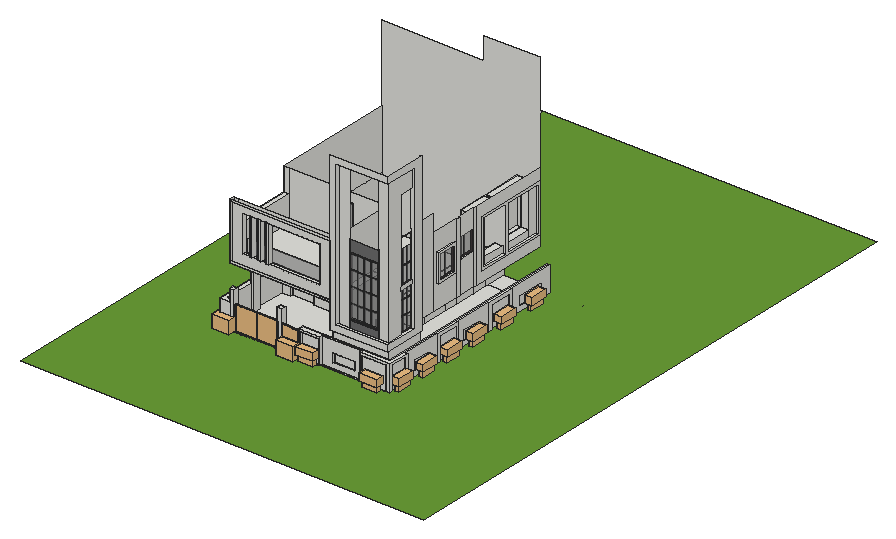
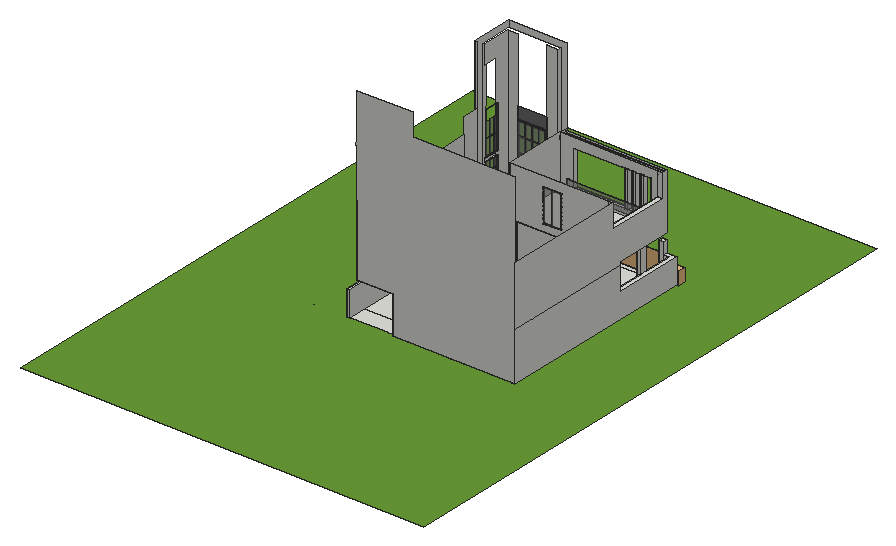
# SketchUp Ruby script. Lengths in inches.
U = 1.inch
M = Sketchup.active_model
def pt(a) = Geom::Point3d.new(a.map { |v| v * U })
def face(e, loops, mat)
  f = e.add_face(loops[0].map { |a| pt(a) })
  loops[1..].each { |l| e.add_face(l.map { |a| pt(a) }).erase! }
  f.material = f.back_material = mat if mat
  f
end
# faces: each face lists its corners as indices into pts; further lists are holes
def faces(e, pts, list, mat = nil) = list.each { |f| face(e, (f[0].is_a?(Array) ? f : [f]).map { |l| l.map { |i| pts[i] } }, mat) }
# xy, xz, yz: faces in a plane at the given z, y or x. An outline is a flat list of corners, or four numbers for a rectangle; further outlines are holes
def ring(l) = l.size == 4 ? [[l[0], l[1]], [l[2], l[1]], [l[2], l[3]], [l[0], l[3]]] : l.each_slice(2).to_a
def flat(e, list, mat, &to3) = list.each { |f| face(e, (f[0].is_a?(Array) ? f : [f]).map { |l| ring(l).map { |u, v| to3.(u, v) } }, mat) }
def xy(e, z, list, mat = nil) = flat(e, list, mat) { |x, y| [x, y, z] }
def xz(e, y, list, mat = nil) = flat(e, list, mat) { |x, z| [x, y, z] }
def yz(e, x, list, mat = nil) = flat(e, list, mat) { |y, z| [x, y, z] }
def lines(e, pts, list) = list.each { |a, b| e.add_line(pt(pts[a]), pt(pts[b])) }
# prism: a flat outline (further loops are holes) pulled along v
def prism(e, loops, v, mat = nil)
  f = face(e, loops, mat); d = Geom::Vector3d.new(v.map { |x| x * U })
  f.pushpull(f.normal.samedirection?(d) ? d.length : -d.length)
end
def box(e, o, s, mat = nil) = prism(e, [[o, [o[0] + s[0], o[1], o[2]], [o[0] + s[0], o[1] + s[1], o[2]], [o[0], o[1] + s[1], o[2]]]], [0, 0, s[2]], mat)
def at(x, y, z, deg = 0) = Geom::Transformation.translation(pt([x, y, z])) * Geom::Transformation.rotation(ORIGIN, Z_AXIS, deg.degrees)
def axes(o, x, y, z) = Geom::Transformation.new([*x, 0, *y, 0, *z, 0, *pt(o).to_a, 1])
def part(name) = M.definitions.add(name)
# library, detail: a bought-in or finely detailed component or shape, given as its bounding box
def library(name, o, s) = part(name).tap { |d| box(d.entities, o, s) }
def detail(e, o, s) = box(e.add_group.entities, o, s)
def put(e, d, t, mat = nil) = e.add_instance(d, t).tap { |i| i.material = mat if mat }
def group(e, t, mat = nil) = e.add_group.tap { |g| g.transformation = t; g.material = mat if mat }.entities
root = M.entities
M.materials.add("Metal Black").color = [38, 38, 38]
M.materials.add("Niraj_Hair_Dark").color = [109, 109, 109]
M.materials.add("[Asphalt New]").color = [67, 60, 62]
M.materials.add("[Grass Dark Green]").color = [106, 157, 55]
M.materials.add("[Translucent Glass Gray]").color = [128, 128, 128]
M.materials["[Translucent Glass Gray]"].alpha = 0.5
c1 = library("Group13",[-203.48,36.63,0],[29.68,67.31,50.64])
c2 = library("Group14",[-195.72,41.78,0],[14.82,56.55,25.56])
c3 = library("Group16",[-203.48,36.63,23.35],[29.68,67.31,27.29])
c4 = part("Group13\#1")
put(c4.entities,c2,at(0,0,0))
put(c4.entities,c3,at(0,0,0))
put(c4.entities,c2,at(-182.87,329.52,-0.08,90))
put(c4.entities,c3,at(-182.87,329.52,-0.08,90))
put(c4.entities,c2,at(-299.3,329.52,-0.08,90))
put(c4.entities,c3,at(-299.3,329.52,-0.08,90))
put(c4.entities,c2,at(-418.4,329.52,-0.08,90))
put(c4.entities,c3,at(-418.4,329.52,-0.08,90))
put(c4.entities,c2,at(-541.23,329.52,-0.08,90))
put(c4.entities,c3,at(-541.23,329.52,-0.08,90))
put(c4.entities,c3,at(-678.71,329.52,-0.08,90))
put(c4.entities,c2,at(-678.71,329.52,-0.08,90))
put(c4.entities,c2,at(-826.74,329.52,-0.08,90))
put(c4.entities,c3,at(-826.74,329.52,-0.08,90))
c5 = part("House+plant_11")
put(c5.entities,c1,axes([-480.16,138.39,0],[0,-3.6636,0],[3.6636,0,0],[0,0,3.6636]))
put(c5.entities,c4,axes([709.84,138.39,0],[0,-3.6636,0],[3.6636,0,0],[0,0,3.6636]))
c6 = part("DOOR12")
g1 = group(c6.entities,at(114.73,28.14,-0.51))
g2 = group(g1,at(0,0,0))
box(g2,[0,0,0],[36,0.5,77.7])
c7 = library("Group\#15",[0.25,0,0],[71.75,3,72.2])
c8 = library("Group\#14",[0.25,0,0],[71.75,3,72.2])
c9 = library("Group\#17",[0,0,0],[42,3,72])
c10 = part("Metal+Gate")
put(c10.entities,c7,axes([-307.79,3014.86,-708.41],[-4,0,0],[0,4,0],[0,0,4.5796]))
put(c10.entities,c8,axes([-307.79,3014.86,-708.41],[4,0,0],[0,4,0],[0,0,4.5796]))
g3 = group(c10.entities,at(-19.79,3008.86,-734.97),"Metal Black")
box(g3,[0,0,13.74],[24,24,343.47])
g4 = group(c10.entities,at(-619.79,3008.86,-734.97),"Metal Black")
box(g4,[0,0,13.74],[24,24,343.47])
put(c10.entities,c9,axes([58.84,3001.49,-721.23],[5.67,0,0],[0,5.67,0],[0,0,4.64321]))
xy(root,0,[[2354.92,2008.02,2385.2,2008.89],[2631.16,2008.02,2652.32,2008.89],[1292.49,2008.89,1428.48,2010.29],[1428.48,2008.89,1484.59,2010.29],[1484.59,2008.89,1540.7,2010.29],
  [1540.7,2008.89,2039.66,2010.29],[2039.66,2008.89,2107.1,2010.29],[2107.1,2008.89,2354.92,2010.29],[2354.92,2008.89,2385.2,2010.29],[2385.2,2008.89,2631.16,2010.29],
  [2631.16,2008.89,2652.32,2010.29],[2652.32,2008.89,3592.26,2010.29],[1226.44,2010.29,1292.49,2076.33],[1292.49,2010.29,1428.48,2076.33],[1428.48,2010.29,2039.66,2076.33],
  [2039.66,2010.29,2107.1,2076.33],[2107.1,2010.29,2354.92,2076.33],[2354.92,2010.29,2354.92,2076.33,3592.26,2076.33,3592.26,2038.35,3249.51,2038.35,3249.51,2010.29,3219.68,2010.29,3219.68,2043.1,2652.32,2043.1,2652.32,2010.29,2631.16,2010.29,2631.16,2022.48,2385.2,2022.48,2385.2,2010.29],[2385.2,2010.29,2631.16,2022.48],[2652.32,2010.29,3219.68,2043.1],
  [3249.51,2010.29,3594.76,2038.35],[3594.76,2010.29,3594.76,2076.33,3592.26,2076.33,3592.26,4870.67,3625.13,4870.67,3625.13,4185.67,3641.13,4185.67,3641.13,4144.69,3621.38,4144.69,3621.38,3821.25,3641.13,3821.25,3641.13,3773.23,3627.94,3773.23,3627.94,3231.42,3641.13,3231.42,3641.13,3197.95,3628.44,3197.95,3628.44,2900.63,3641.13,2900.63,3641.13,2868.54,3630.25,2868.54,3630.25,2319.96,3647.19,2319.96,3647.19,2285.03,3629.25,2285.03,3629.25,2048.41,3647.19,2048.41,3647.19,2010.29],[3592.26,2038.35,3594.76,2076.33],[1226.44,2076.33,1226.44,4883.98,2686.29,4883.98,2686.29,3028.71,1755,3028.71,1755,3092.96,1428.32,3092.96,1428.32,3028.71,1292.49,3028.71,1292.49,2577.21,1338.09,2577.21,1338.09,2475.3,1292.49,2475.3,1292.49,2076.33],[1292.49,2076.33,1292.49,2475.3,1338.09,2475.3,1338.09,2577.21,1292.49,2577.21,1292.49,3028.71,1428.32,3028.71,1428.32,3092.96,1755,3092.96,1755,3028.71,2686.29,3028.71,2686.29,2203.14,3472.07,2203.14,3472.07,2760.56,2969.57,2760.56,2969.57,3198.71,2952.76,3198.71,2952.76,3451.83,2969.57,3451.83,2969.57,3827.1875,2935.26,3827.1875,2935.26,4052.1875,2969.57,4052.1875,2969.57,4325.15,2934.2,4325.15,2934.2,4554.96,2969.57,4554.96,2969.57,4598.11,3592.26,4598.11,3592.26,2076.33],
  [2686.29,2203.14,2686.29,3073.14,2969.57,3073.14,2969.57,2760.56,3472.07,2760.56,3472.07,2203.14],[2686.29,3073.14,2686.29,4883.98,2969.57,4883.98,2969.57,4554.96,2934.2,4554.96,2934.2,4325.15,2969.57,4325.15,2969.57,4052.1875,2935.26,4052.1875,2935.26,3827.1875,2969.57,3827.1875,2969.57,3451.83,2952.76,3451.83,2952.76,3198.71,2969.57,3198.71,2969.57,3073.14],[2969.57,4598.11,3592.26,4870.67]])
xy(root,0,[[[0,0,5734.0625,8045.6875],[1292.49,2008.89,2354.92,2008.89,2354.92,2010.29,2385.2,2010.29,2385.2,2008.89,2631.16,2008.89,2631.16,2010.29,2652.32,2010.29,2652.32,2008.89,3592.26,2008.89,3592.26,2010.29,3647.19,2010.29,3647.19,2048.41,3629.25,2048.41,3629.25,2285.03,3647.19,2285.03,3647.19,2319.96,3630.25,2319.96,3630.25,2868.54,3641.13,2868.54,3641.13,2900.63,3628.44,2900.63,3628.44,3197.95,3641.13,3197.95,3641.13,3231.42,3627.94,3231.42,3627.94,3773.23,3641.13,3773.23,3641.13,3821.25,3621.38,3821.25,3621.38,4144.69,3641.13,4144.69,3641.13,4185.67,3625.13,4185.67,3625.13,4870.67,2969.57,4870.67,2969.57,4883.98,1226.44,4883.98,1226.44,2010.29,1292.49,2010.29],[2354.92,2008.02,2385.2,2008.89],[2631.16,2008.02,2652.32,2008.89]]],"[Grass Dark Green]")
xy(root,52.04,[[3572.25,3336.62,3627.94,3643.37]])
xy(root,59.12,[[3584.75,2463.8125,3630.25,2744.9375]])
xy(root,69.24,[[3608.5,4331.26,3625.13,4732.32]])
xy(root,69.81,[[2815.04,2043.1,3114.47,2132.41]])
xy(root,204.24,[[2815.04,2043.1,3114.47,2132.41]])
xy(root,207.06,[[3608.5,4331.26,3625.13,4732.32]])
xy(root,207.31,[[3584.75,2463.8125,3630.25,2744.9375]])
xy(root,207.91,[[3572.25,3336.62,3627.94,3643.37]])
xy(root,323.4375,[[3621.38,3821.25,3641.13,4144.69]])
xy(root,329.125,[[3628.44,2900.63,3641.13,3197.95]])
xy(root,333.04,[[3249.51,2010.29,3594.76,2038.35]])
xy(root,334.16,[[2385.2,2008.02,2631.16,2022.48]])
xy(root,338.5625,[[3629.25,2048.41,3647.19,2285.03]])
xy(root,356.375,[[1226.44,2010.29,1363.79,2010.29,1363.79,2076.33,1292.49,2076.33,1292.49,3028.71,1226.44,3028.71]])
xy(root,362.875,[[2354.92,2008.02,2652.32,2008.02,2652.32,2043.1,2637.26,2043.1,2637.26,2076.33,2354.92,2076.33],[3219.68,2010.29,3647.19,2010.29,3647.19,2319.96,3592.26,2319.96,3592.26,2076.33,2637.26,2076.33,2637.26,2043.1,3219.68,2043.1],[3592.26,2319.96,3630.25,2319.96,3630.25,2868.54,3641.13,2868.54,3641.13,3231.42,3627.94,3231.42,3627.94,3773.23,3641.13,3773.23,3641.13,4185.67,3625.13,4185.67,3625.13,4870.67,3592.26,4870.67]])
xy(root,379.75,[[2949.82,3541.14,2969.57,3628.45]])
xy(root,402.55,[[2686.29,2150.08,3502.39,2203.14],[3472.07,2203.14,3502.39,2760.56]])
xy(root,454.11,[[2952.76,3198.71,2969.57,3451.83],[2935.26,3827.1875,2969.57,4052.1875]])
xy(root,454.6875,[[2934.2,4325.15,2969.57,4554.96]])
xy(root,467.36,[[2949.82,3541.14,2969.57,3628.45]])
xy(root,489.56,[[2759.375,2150.08,3502.39,2150.08,3502.39,2203.14,3331.43,2203.14,3331.43,2198.52,2926.88,2198.52,2926.88,2203.14,2759.375,2203.14],[3472.07,2203.14,3502.39,2203.14,3502.39,2625.31,3456.14,2625.31,3456.14,2414.23,3472.07,2414.23]])
xy(root,522.8125,[[1363.79,2010.29,1428.48,2076.33],[2039.66,2010.29,2107.1,2076.33]])
xy(root,535.62,[[2969.57,2760.56,2969.57,4883.98,3472.07,4883.98,3472.07,3749.47,3483.14,3749.47,3483.14,3710.59,3467.64,3710.59,3467.64,3450.16,3483.14,3450.16,3483.14,3408.39,3472.07,3408.39,3472.07,2760.56]])
xy(root,606.87,[[2938.7,2198.52,3319.62,2223.02]],"[Asphalt New]")
xy(root,641.5,[[1428.32,3028.71,1755,3092.96]])
xy(root,689.25,[[1292.49,2475.3,1338.09,2577.21]])
xy(root,689.32,[[3472.07,3842.77,3484.89,4883.98]])
xy(root,712.75,[[3175.57,3866.2,3330.23,4265.09],[3445.71,3866.2,3484.89,4265.09],[3175.57,4299.68,3330.23,4860.56],[3445.71,4299.68,3484.89,4860.56]])
xy(root,730.9375,[[1226.44,2185.52,2686.29,3028.71]])
xy(root,751.625,[[1247.13,2185.52,2665.6,2203.14]])
xy(root,805.62,[[3330.23,3938.51,3445.71,4265.09],[3330.23,4299.68,3445.71,4735.52]])
xy(root,831.12,[[[1302.24,2260.63,2686.29,3149.5625],[1380.99,2322.26,2541.12,2326.6]]])
xy(root,880.73,[[3472.07,3051.17,3505.51,3357.79]])
xy(root,885.11,[[1394.43,2203.14,1496.38,2260.63],[1496.38,2203.14,1535.24,2260.63],[1535.24,2203.14,1613.13,2260.63],[1613.13,2203.14,1651.99,2260.63],[1651.99,2203.14,1726.63,2260.63],
  [1726.63,2203.14,1765.49,2260.63],[1765.49,2203.14,2498.31,2260.63]])
xy(root,900.6875,[[3472.07,3071.125,3505.51,3337.83]])
xy(root,986.66,[[3445.7,3450.16,3467.64,3710.59]])
xy(root,1022.3,[[1380.99,2322.26,2541.12,2326.6]])
xy(root,1049.9,[[3456.14,2414.23,3472.07,2625.31]])
xy(root,1102.3125,[[3456.14,2414.23,3472.07,2625.31]])
xy(root,1204.68,[[1226.44,2260.63,1302.24,3149.5625]])
xy(root,1252.83,[[3472.07,3071.125,3505.51,3337.83]])
xy(root,1272.79,[[3472.07,3051.17,3505.51,3357.79]])
xy(root,1279.12,[[3445.7,3450.16,3467.64,3710.59]])
xy(root,1325.25,[[3330.23,4735.52,3445.71,4860.56]])
xy(root,1352.49,[[3175.57,3866.2,3175.57,4265.09,3484.89,4265.09,3484.89,3866.2,3445.71,3866.2,3445.71,3938.51,3330.23,3938.51,3330.23,3866.2],[3175.57,4265.09,3484.89,4299.68],[3175.57,4299.68,3484.89,4860.56]])
xy(root,1375.92,[[3472.07,3842.77,3484.89,4883.98]])
xy(root,1408.74,[[1394.43,2203.14,1496.38,2260.63],[1496.38,2203.14,1535.24,2260.63],[1535.24,2203.14,1613.13,2260.63],[1613.13,2203.14,1651.99,2260.63],[1651.99,2203.14,1726.63,2260.63],
  [1726.63,2203.14,1765.49,2260.63],[1765.49,2203.14,2498.31,2260.63]])
xy(root,1440.24,[[2938.7,2198.52,3319.62,2223.02]],"[Asphalt New]")
xz(root,2008.02,[[2354.92,0,2385.2,0,2385.2,334.16,2631.16,334.16,2631.16,0,2652.32,0,2652.32,362.875,2354.92,362.875]])
xz(root,2010.29,[[1226.44,0,1363.79,356.375],[1363.79,0,1428.48,522.8125],[2039.66,0,2107.1,522.8125],[3219.68,0,3249.51,0,3249.51,333.04,3594.76,333.04,3594.76,0,3647.19,0,3647.19,362.875,3219.68,362.875],[3249.51,0,3594.76,333.04]])
xz(root,2022.48,[[2385.2,0,2631.16,334.16]])
xz(root,2038.35,[[3249.51,0,3594.76,333.04]])
xz(root,2043.1,[[[2652.32,0,3219.68,362.875],[2815.04,69.81,3114.47,204.24]]])
xz(root,2048.41,[[3629.25,0,3647.19,338.5625]])
xz(root,2076.33,[[1292.49,0,1363.79,356.375],[1363.79,0,1428.48,522.8125],[2039.66,0,2107.1,522.8125],[2354.92,0,2637.26,362.875],[2637.26,0,3592.26,362.875],
  [3592.26,0,3594.76,362.875]])
xz(root,2132.41,[[2815.04,69.81,3114.47,204.24]])
xz(root,2150.08,[[2686.29,402.55,3502.39,402.55,3502.39,489.56,2759.375,489.56,2759.375,2542.29,3502.39,2542.29,3502.39,2628.8125,2686.29,2628.8125]])
xz(root,2185.52,[[[1226.44,730.9375,2686.29,1537],[1247.13,751.625,2665.6,1516.31]]])
xz(root,2198.52,[[2926.88,489.56,3331.43,595.05],[2926.88,1452.06,3331.43,1617.11]],"Niraj_Hair_Dark")
xz(root,2198.52,[[2926.88,595.05,3331.43,595.05,3331.43,1452.06,3236.17,1452.06,3236.17,1440.24,3319.62,1440.24,3319.62,606.87,2938.7,606.87,2938.7,1440.24,3033.28,1440.24,3033.28,1452.06,2926.88,1452.06],[3033.28,606.87,3041.55,802.14],[3129.16,606.87,3135.04,802.14],[3227.98,606.87,3236.17,802.14],[2938.7,802.14,3033.28,811.5],
  [3033.28,802.14,3041.55,811.5],[3041.55,802.14,3129.16,811.5],[3129.16,802.14,3135.04,811.5],[3135.04,802.14,3227.98,811.5],[3227.98,802.14,3236.17,811.5],
  [3236.17,802.14,3319.62,811.5],[3033.28,811.5,3041.55,1016.13],[3129.16,811.5,3135.04,1016.13],[3227.98,811.5,3236.17,1016.13],[2938.7,1016.13,3033.28,1023.55],
  [3033.28,1016.13,3041.55,1023.55],[3041.55,1016.13,3129.16,1023.55],[3129.16,1016.13,3135.04,1023.55],[3135.04,1016.13,3227.98,1023.55],[3227.98,1016.13,3236.17,1023.55],
  [3236.17,1016.13,3319.62,1023.55],[3033.28,1023.55,3041.55,1231.9],[3129.16,1023.55,3135.04,1231.9],[3227.98,1023.55,3236.17,1231.9],[2938.7,1231.9,3033.28,1239.71],
  [3033.28,1231.9,3041.55,1239.71],[3041.55,1231.9,3129.16,1239.71],[3129.16,1231.9,3135.04,1239.71],[3135.04,1231.9,3227.98,1239.71],[3227.98,1231.9,3236.17,1239.71],
  [3236.17,1231.9,3319.62,1239.71],[3033.28,1239.71,3041.55,1440.24],[3129.16,1239.71,3135.04,1440.24],[3227.98,1239.71,3236.17,1440.24],[3033.28,1440.24,3041.55,1452.06],
  [3041.55,1440.24,3129.16,1452.06],[3129.16,1440.24,3135.04,1452.06],[3135.04,1440.24,3227.98,1452.06],[3227.98,1440.24,3236.17,1452.06]],"[Asphalt New]")
xz(root,2198.52,[[2938.7,606.87,3033.28,802.14],[3041.55,606.87,3129.16,802.14],[3135.04,606.87,3227.98,802.14],[3236.17,606.87,3319.62,802.14],[2938.7,811.5,3033.28,1016.13],
  [3041.55,811.5,3129.16,1016.13],[3135.04,811.5,3227.98,1016.13],[3236.17,811.5,3319.62,1016.13],[2938.7,1023.55,3033.28,1231.9],[3041.55,1023.55,3129.16,1231.9],
  [3135.04,1023.55,3227.98,1231.9],[3236.17,1023.55,3319.62,1231.9],[2938.7,1239.71,3033.28,1440.24],[3041.55,1239.71,3129.16,1440.24],[3135.04,1239.71,3227.98,1440.24],
  [3236.17,1239.71,3319.62,1440.24]],"[Translucent Glass Gray]")
xz(root,2203.14,[[2686.29,0,3472.07,402.55],[2759.375,489.56,2926.88,2542.29],[3331.43,489.56,3472.07,2542.29],[[1247.13,751.625,2665.6,1516.31],[1394.43,885.11,2498.31,1408.74]],[1496.38,885.11,1535.24,1408.74],
  [1613.13,885.11,1651.99,1408.74],[1726.63,885.11,1765.49,1408.74]])
xz(root,2223.02,[[2938.7,606.87,3319.62,1440.24]],"[Translucent Glass Gray]")
xz(root,2260.63,[[[1302.24,831.12,2686.29,1537],[1394.43,885.11,2498.31,1408.74]],[1496.38,885.11,1535.24,1408.74],[1613.13,885.11,1651.99,1408.74],[1726.63,885.11,1765.49,1408.74],[1226.44,1204.68,1302.24,1537]])
xz(root,2285.03,[[3629.25,0,3647.19,338.5625]])
xz(root,2319.96,[[3630.25,0,3647.19,362.875]])
xz(root,2326.6,[[1380.99,831.12,2541.12,1022.3]],"[Translucent Glass Gray]")
xz(root,2414.23,[[3456.14,489.56,3472.07,1049.9],[3456.14,1102.3125,3472.07,1715.07]])
xz(root,2463.8125,[[3584.75,59.12,3630.25,207.31]])
xz(root,2475.3,[[1292.49,0,1338.09,689.25]])
xz(root,2577.21,[[1292.49,0,1338.09,689.25]])
xz(root,2625.31,[[3456.14,489.56,3502.39,489.56,3502.39,2542.29,3472.07,2542.29,3472.07,2280.66,3456.14,2280.66,3456.14,1763.16,3472.07,1763.16,3472.07,1715.07,3456.14,1715.07,3456.14,1102.3125,3472.07,1102.3125,3472.07,1049.9,3456.14,1049.9]])
xz(root,2744.9375,[[3584.75,59.12,3630.25,207.31]])
xz(root,2760.56,[[2969.57,0,3472.07,402.55],[2969.57,402.55,2969.57,535.62,3472.07,535.62,3472.07,2628.8125,3502.39,2628.8125,3502.39,402.55]])
xz(root,2868.54,[[3630.25,0,3641.13,362.875]])
xz(root,2900.63,[[3628.44,0,3641.13,329.125]])
xz(root,3028.71,[[1292.49,0,1428.32,0,1428.32,641.5,1755,641.5,1755,0,2686.29,0,2686.29,730.9375,1226.44,730.9375,1226.44,356.375,1292.49,356.375]])
xz(root,3051.17,[[3472.07,880.73,3505.51,1272.79]])
xz(root,3071.125,[[3472.07,900.6875,3505.51,1252.83]])
xz(root,3092.96,[[1428.32,0,1755,641.5]])
xz(root,3149.5625,[[[1302.24,831.12,2686.29,1537],[1949.51,924.7,2225.45,1411.26]],[1226.44,1204.68,1302.24,1537]])
xz(root,3149.5625,[[[1949.51,924.7,2225.45,1411.26],[1960.18,935.37,2214.77,1400.59]],[2087.48,935.37,2098.12,1400.59]],"[Asphalt New]")
xz(root,3149.5625,[[1960.18,935.37,2087.48,1400.59],[2098.12,935.37,2214.77,1400.59]],"[Translucent Glass Gray]")
xz(root,3197.95,[[3628.44,0,3641.13,329.125]])
xz(root,3198.71,[[2952.76,0,2969.57,454.11]])
xz(root,3231.42,[[3627.94,0,3641.13,362.875]])
xz(root,3336.62,[[3572.25,52.04,3627.94,207.91]])
xz(root,3337.83,[[3472.07,900.6875,3505.51,1252.83]])
xz(root,3357.79,[[3472.07,880.73,3505.51,1272.79]])
xz(root,3408.39,[[3472.07,535.62,3483.14,1540.5]])
xz(root,3450.16,[[3467.64,535.62,3467.64,986.66,3445.7,986.66,3445.7,1279.12,3467.64,1279.12,3467.64,1540.5,3483.14,1540.5,3483.14,535.62]])
xz(root,3451.83,[[2952.76,0,2969.57,454.11]])
xz(root,3541.14,[[2949.82,379.75,2969.57,467.36]])
xz(root,3628.45,[[2949.82,379.75,2969.57,467.36]])
xz(root,3643.37,[[3572.25,52.04,3627.94,207.91]])
xz(root,3710.59,[[3467.64,535.62,3483.14,535.62,3483.14,1540.5,3467.64,1540.5,3467.64,1279.12,3445.7,1279.12,3445.7,986.66,3467.64,986.66]])
xz(root,3749.47,[[3472.07,535.62,3483.14,1540.5]])
xz(root,3773.23,[[3627.94,0,3641.13,362.875]])
xz(root,3821.25,[[3621.38,0,3641.13,323.4375]])
xz(root,3827.1875,[[2935.26,0,2969.57,454.11]])
xz(root,3842.77,[[3472.07,689.32,3484.89,1375.92]])
xz(root,3866.2,[[3175.57,712.75,3330.23,1352.49],[3445.71,712.75,3484.89,1352.49]])
xz(root,3938.51,[[3330.23,805.62,3445.71,1352.49]])
xz(root,4052.1875,[[2935.26,0,2969.57,454.11]])
xz(root,4144.69,[[3621.38,0,3641.13,323.4375]])
xz(root,4185.67,[[3625.13,0,3641.13,362.875]])
xz(root,4265.09,[[3175.57,712.75,3330.23,712.75,3330.23,805.62,3445.71,805.62,3445.71,712.75,3484.89,712.75,3484.89,1352.49,3175.57,1352.49]])
xz(root,4299.68,[[3175.57,712.75,3175.57,1352.49,3484.89,1352.49,3484.89,712.75,3445.71,712.75,3445.71,805.62,3330.23,805.62,3330.23,712.75]])
xz(root,4325.15,[[2934.2,0,2969.57,454.6875]])
xz(root,4331.26,[[3608.5,69.24,3625.13,207.06]])
xz(root,4554.96,[[2934.2,0,2969.57,454.6875]])
xz(root,4732.32,[[3608.5,69.24,3625.13,207.06]])
xz(root,4735.52,[[3330.23,805.62,3445.71,1325.25]])
xz(root,4860.56,[[3175.57,712.75,3330.23,712.75,3330.23,1325.25,3445.71,1325.25,3445.71,712.75,3484.89,712.75,3484.89,1352.49,3175.57,1352.49]])
xz(root,4870.67,[[3592.26,0,3625.13,362.875]])
xz(root,4883.98,[[1226.44,0,1226.44,2628.8125,2686.29,2628.8125,2686.29,2946.875,3472.07,2946.875,3472.07,2269.31,3494.39,2269.31,3494.39,2242.5,3472.07,2242.5,3472.07,1375.92,3484.89,1375.92,3484.89,689.32,3472.07,689.32,3472.07,535.62,2969.57,535.62,2969.57,0]])
yz(root,1226.44,[[2010.29,0,2010.29,356.375,3028.71,356.375,3028.71,689.25,4883.98,689.25,4883.98,0],[3028.71,689.25,3028.71,730.9375,2185.52,730.9375,2185.52,1537,2260.63,1537,2260.63,1204.68,3149.5625,1204.68,3149.5625,1537,4883.98,1537,4883.98,689.25]])
yz(root,1247.13,[[2185.52,751.625,2203.14,1516.31]])
yz(root,1292.49,[[2076.33,0,2475.3,356.375],[2577.21,0,3028.71,356.375],[2475.3,356.375,2577.21,689.25]])
yz(root,1302.24,[[2260.63,831.12,3149.5625,1204.68]])
yz(root,1338.09,[[2475.3,0,2577.21,689.25]])
yz(root,1363.79,[[2010.29,356.375,2076.33,522.8125]])
yz(root,1380.99,[[2322.26,831.12,2326.6,1022.3]])
yz(root,1394.43,[[2203.14,885.11,2260.63,1408.74]])
yz(root,1428.32,[[3028.71,0,3092.96,641.5]])
yz(root,1428.48,[[2010.29,0,2076.33,522.8125]])
yz(root,1496.38,[[2203.14,885.11,2260.63,1408.74]])
yz(root,1535.24,[[2203.14,885.11,2260.63,1408.74]])
yz(root,1613.13,[[2203.14,885.11,2260.63,1408.74]])
yz(root,1651.99,[[2203.14,885.11,2260.63,1408.74]])
yz(root,1726.63,[[2203.14,885.11,2260.63,1408.74]])
yz(root,1755,[[3028.71,0,3092.96,641.5]])
yz(root,1765.49,[[2203.14,885.11,2260.63,1408.74]])
yz(root,2039.66,[[2010.29,0,2076.33,522.8125]])
yz(root,2107.1,[[2010.29,0,2076.33,522.8125]])
yz(root,2354.92,[[2008.02,0,2076.33,362.875]])
yz(root,2385.2,[[2008.02,0,2022.48,334.16]])
yz(root,2498.31,[[2203.14,885.11,2260.63,1408.74]])
yz(root,2541.12,[[2322.26,831.12,2326.6,1022.3]])
yz(root,2631.16,[[2008.02,0,2022.48,334.16]])
yz(root,2652.32,[[2008.02,0,2043.1,362.875]])
yz(root,2665.6,[[2185.52,751.625,2203.14,1516.31]])
yz(root,2686.29,[[2203.14,0,2203.14,402.55,2150.08,402.55,2150.08,730.9375,3028.71,730.9375,3028.71,0],[2150.08,730.9375,2185.52,1537],[2185.52,730.9375,2185.52,1537,2260.63,1537,2203.14,730.9375],[2260.63,831.12,3149.5625,1537]])
yz(root,2759.375,[[2150.08,489.56,2203.14,2542.29]])
yz(root,2815.04,[[2043.1,69.81,2132.41,204.24]])
yz(root,2926.88,[[2198.52,489.56,2203.14,595.05],[2198.52,1452.06,2203.14,1617.11]],"Niraj_Hair_Dark")
yz(root,2926.88,[[2198.52,595.05,2203.14,1452.06]],"[Asphalt New]")
yz(root,2934.2,[[4325.15,0,4554.96,454.6875]])
yz(root,2935.26,[[3827.1875,0,4052.1875,454.11]])
yz(root,2938.7,[[2198.52,606.87,2223.02,1440.24]],"[Asphalt New]")
yz(root,2949.82,[[3541.14,379.75,3628.45,467.36]],"[Translucent Glass Gray]")
yz(root,2952.76,[[3198.71,0,3451.83,454.11]])
yz(root,2969.57,[[[2760.56,0,3198.71,0,3198.71,454.11,3451.83,454.11,3451.83,0,3827.1875,0,3827.1875,454.11,4052.1875,454.11,4052.1875,0,4325.15,0,4325.15,454.6875,4554.96,454.6875,4554.96,0,4883.98,0,4883.98,535.62,2760.56,535.62],[3541.14,379.75,3628.45,467.36]]])
yz(root,3114.47,[[2043.1,69.81,2132.41,204.24]])
yz(root,3175.57,[[3866.2,712.75,4265.09,1352.49],[4299.68,712.75,4860.56,1352.49]])
yz(root,3219.68,[[2010.29,0,2043.1,362.875]])
yz(root,3249.51,[[2010.29,0,2038.35,333.04]])
yz(root,3319.62,[[2198.52,606.87,2223.02,1440.24]],"[Asphalt New]")
yz(root,3330.23,[[3866.2,712.75,3938.51,1352.49],[3938.51,712.75,4265.09,805.62],[4299.68,712.75,4735.52,805.62],[4735.52,712.75,4860.56,1325.25]])
yz(root,3331.43,[[2198.52,489.56,2203.14,595.05],[2198.52,1452.06,2203.14,1617.11]],"Niraj_Hair_Dark")
yz(root,3331.43,[[2198.52,595.05,2203.14,1452.06]],"[Asphalt New]")
yz(root,3445.7,[[[3450.16,986.66,3710.59,1279.12],[3462.85,999.35,3697.89,1266.43]],[3569.45,999.35,3580.37,1266.43]],"[Asphalt New]")
yz(root,3445.7,[[3462.85,999.35,3569.45,1266.43],[3580.37,999.35,3697.89,1266.43]],"[Translucent Glass Gray]")
yz(root,3445.71,[[3866.2,712.75,3938.51,1352.49],[3938.51,712.75,4265.09,805.62],[4299.68,712.75,4735.52,805.62],[4735.52,712.75,4860.56,1325.25]])
yz(root,3456.14,[[[2414.23,489.56,2625.31,1049.9],[2421.72,497.05,2617.8125,1042.41]],[2477.95,497.05,2483.89,693.06],[2550.85,497.05,2556.97,693.06],[2421.72,693.06,2477.95,700.05],[2477.95,693.06,2483.89,700.05],
  [2483.89,693.06,2550.85,700.05],[2550.85,693.06,2556.97,700.05],[2556.97,693.06,2617.8125,700.05],[2477.95,700.05,2483.89,903.05],[2550.85,700.05,2556.97,903.05],
  [2421.72,903.05,2477.95,911.17],[2477.95,903.05,2483.89,911.17],[2483.89,903.05,2550.85,911.17],[2550.85,903.05,2556.97,911.17],[2556.97,903.05,2617.8125,911.17],
  [2477.95,911.17,2483.89,1042.41],[2550.85,911.17,2556.97,1042.41],[[2414.23,1102.3125,2625.31,1715.07],[2420.15,1108.24,2619.39,1709.15]],[2466.95,1108.24,2475.41,1334.36],[2547.4,1108.24,2555.61,1334.36],
  [2420.15,1334.36,2466.95,1343.63],[2466.95,1334.36,2475.41,1343.63],[2475.41,1334.36,2547.4,1343.63],[2547.4,1334.36,2555.61,1343.63],[2555.61,1334.36,2619.39,1343.63],
  [2466.95,1343.63,2475.41,1560.48],[2547.4,1343.63,2555.61,1560.48]],"[Asphalt New]")
yz(root,3456.14,[[2421.72,497.05,2477.95,693.06],[2483.89,497.05,2550.85,693.06],[2556.97,497.05,2617.8125,693.06],[2421.72,700.05,2477.95,903.05],[2483.89,700.05,2550.85,903.05],
  [2556.97,700.05,2617.8125,903.05],[2421.72,911.17,2477.95,1042.41],[2483.89,911.17,2550.85,1042.41],[2556.97,911.17,2617.8125,1042.41],[2420.15,1108.24,2466.95,1334.36],
  [2475.41,1108.24,2547.4,1334.36],[2555.61,1108.24,2619.39,1334.36],[2420.15,1343.63,2466.95,1560.48],[2475.41,1343.63,2547.4,1560.48],[2555.61,1343.63,2619.39,1560.48]],"[Translucent Glass Gray]")
yz(root,3467.64,[[3450.16,535.62,3710.59,986.66],[3450.16,1279.12,3710.59,1540.5]])
yz(root,3472.07,[[2203.14,0,2760.56,402.55],[2203.14,489.56,2414.23,489.56,2414.23,2280.66,2625.31,2280.66,2625.31,2542.29,2203.14,2542.29],[2760.56,535.62,2984.77,1781.04],[[2984.77,535.62,3408.39,1540.5],[3051.17,880.73,3357.79,1272.79]],[3749.47,535.62,4883.98,535.62,4883.98,689.32,3842.77,689.32,3842.77,1375.92,4883.98,1375.92,4883.98,1540.5,3749.47,1540.5],
  [2414.23,1049.9,2625.31,1102.3125]])
yz(root,3472.07,[[[3071.125,900.6875,3337.83,1252.83],[3075.24,904.8,3333.71,1248.72]],[3204.48,904.8,3211.42,1248.72]],"[Asphalt New]")
yz(root,3472.07,[[3075.24,904.8,3204.48,1248.72],[3211.42,904.8,3333.71,1248.72]],"[Translucent Glass Gray]")
yz(root,3483.14,[[3408.39,535.62,3450.16,1540.5],[3710.59,535.62,3749.47,1540.5]])
yz(root,3484.89,[[[3842.77,689.32,4883.98,1375.92],[4299.68,712.75,4860.56,1352.49],[3866.2,712.75,4265.09,1352.49]]])
yz(root,3502.39,[[2150.08,402.55,2760.56,402.55,2760.56,2628.8125,2150.08,2628.8125,2150.08,2542.29,2625.31,2542.29,2625.31,489.56,2150.08,489.56]])
yz(root,3505.51,[[[3051.17,880.73,3357.79,1272.79],[3071.125,900.6875,3337.83,1252.83]]])
yz(root,3572.25,[[3336.62,52.04,3643.37,207.91]])
yz(root,3584.75,[[2463.8125,59.12,2744.9375,207.31]])
yz(root,3592.26,[[2076.33,0,4870.67,362.875]])
yz(root,3594.76,[[2010.29,0,2038.35,333.04]])
yz(root,3608.5,[[4331.26,69.24,4732.32,207.06]])
yz(root,3621.38,[[3821.25,0,4144.69,323.4375]])
yz(root,3625.13,[[[4185.67,0,4870.67,362.875],[4331.26,69.24,4732.32,207.06]]])
yz(root,3627.94,[[[3231.42,0,3773.23,362.875],[3336.62,52.04,3643.37,207.91]]])
yz(root,3628.44,[[2900.63,0,3197.95,329.125]])
yz(root,3629.25,[[2048.41,0,2285.03,338.5625]])
yz(root,3630.25,[[[2319.96,0,2868.54,362.875],[2463.8125,59.12,2744.9375,207.31]]])
yz(root,3641.13,[[2868.54,0,2900.63,0,2900.63,329.125,3197.95,329.125,3197.95,0,3231.42,0,3231.42,362.875,2868.54,362.875],[3773.23,0,3821.25,0,3821.25,323.4375,4144.69,323.4375,4144.69,0,4185.67,0,4185.67,362.875,3773.23,362.875]])
yz(root,3647.19,[[2010.29,0,2048.41,0,2048.41,338.5625,2285.03,338.5625,2285.03,0,2319.96,0,2319.96,362.875,2010.29,362.875]])
p = [[2686.29,3073.14,689.25],[2686.29,3268.14,689.25],[4093.07,4870.67,0],[4093.07,4883.98,0]]
lines(root,p,[[0,1],[2,3]])
put(root,c5,at(1537.08,1133.93,0))
put(root,c5,at(2463.45,1112.93,0))
put(root,c6,axes([388.42,2824.85,4.21],[9.064,0,0],[0,8.24,0],[0,0,8.24]))
put(root,c6,axes([3134.98,3018.56,3],[0,7.04822,0],[-5.87842,0,0],[0,0,5.87842]))
put(root,c6,axes([3134.98,3516.52,3],[0,7.04822,0],[-5.87842,0,0],[0,0,5.87842]))
put(root,c10,at(2048.27,-994.03,721.23))
put(root,c6,axes([3137.92,2390.08,3],[0,7.04822,0],[-5.87842,0,0],[0,0,5.87842]))
